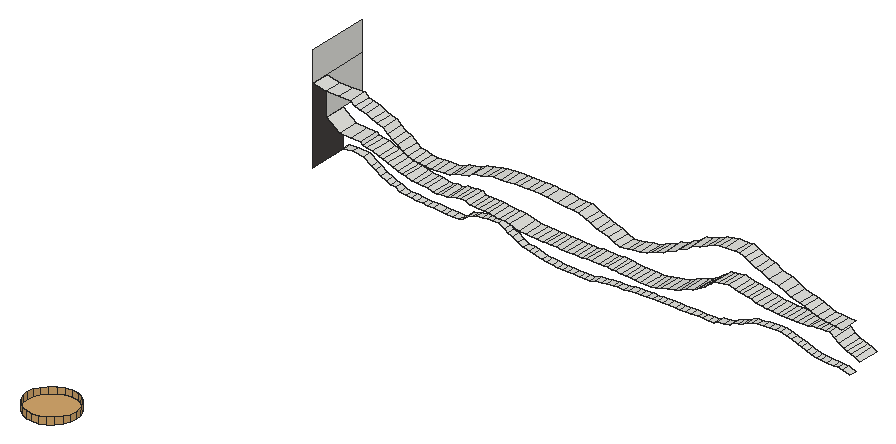
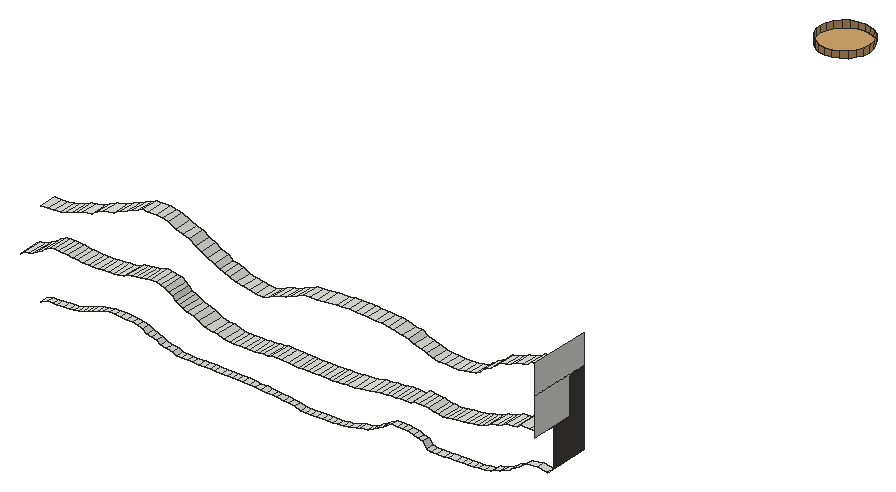
# SketchUp Ruby script. Lengths in inches.
U = 1.inch
M = Sketchup.active_model
def pt(a) = Geom::Point3d.new(a.map { |v| v * U })
def face(e, loops, mat)
  f = e.add_face(loops[0].map { |a| pt(a) })
  loops[1..].each { |l| e.add_face(l.map { |a| pt(a) }).erase! }
  f.material = f.back_material = mat if mat
  f
end
# faces: each face lists its corners as indices into pts; further lists are holes
def faces(e, pts, list, mat = nil) = list.each { |f| face(e, (f[0].is_a?(Array) ? f : [f]).map { |l| l.map { |i| pts[i] } }, mat) }
# xy, xz, yz: faces in a plane at the given z, y or x. An outline is a flat list of corners, or four numbers for a rectangle; further outlines are holes
def ring(l) = l.size == 4 ? [[l[0], l[1]], [l[2], l[1]], [l[2], l[3]], [l[0], l[3]]] : l.each_slice(2).to_a
def flat(e, list, mat, &to3) = list.each { |f| face(e, (f[0].is_a?(Array) ? f : [f]).map { |l| ring(l).map { |u, v| to3.(u, v) } }, mat) }
def xy(e, z, list, mat = nil) = flat(e, list, mat) { |x, y| [x, y, z] }
def xz(e, y, list, mat = nil) = flat(e, list, mat) { |x, z| [x, y, z] }
def yz(e, x, list, mat = nil) = flat(e, list, mat) { |y, z| [x, y, z] }
def lines(e, pts, list) = list.each { |a, b| e.add_line(pt(pts[a]), pt(pts[b])) }
# prism: a flat outline (further loops are holes) pulled along v
def prism(e, loops, v, mat = nil)
  f = face(e, loops, mat); d = Geom::Vector3d.new(v.map { |x| x * U })
  f.pushpull(f.normal.samedirection?(d) ? d.length : -d.length)
end
def box(e, o, s, mat = nil) = prism(e, [[o, [o[0] + s[0], o[1], o[2]], [o[0] + s[0], o[1] + s[1], o[2]], [o[0], o[1] + s[1], o[2]]]], [0, 0, s[2]], mat)
def at(x, y, z, deg = 0) = Geom::Transformation.translation(pt([x, y, z])) * Geom::Transformation.rotation(ORIGIN, Z_AXIS, deg.degrees)
def axes(o, x, y, z) = Geom::Transformation.new([*x, 0, *y, 0, *z, 0, *pt(o).to_a, 1])
def part(name) = M.definitions.add(name)
# library, detail: a bought-in or finely detailed component or shape, given as its bounding box
def library(name, o, s) = part(name).tap { |d| box(d.entities, o, s) }
def detail(e, o, s) = box(e.add_group.entities, o, s)
def put(e, d, t, mat = nil) = e.add_instance(d, t).tap { |i| i.material = mat if mat }
def group(e, t, mat = nil) = e.add_group.tap { |g| g.transformation = t; g.material = mat if mat }.entities
root = M.entities
M.materials.add("[Field Square Tile]").color = [211, 167, 108]
M.materials.add("[Granite Tile]1").color = [68, 65, 63]
xy(root,237.65,[[282.08,565.74,282.77,566.68],[282.77,565.74,283.39,566.68]])
xy(root,238.33,[[291.18,565.74,291.73,566.68],[291.73,565.74,292.41,566.68]])
xy(root,238.34,[[293.09,565.74,294.02,566.68],[294.02,565.74,294.51,566.68],[294.51,565.74,295.27,566.68],[295.27,565.74,295.9,566.68],[295.9,565.74,296.65,566.68],
  [296.65,565.74,297.27,566.68],[297.27,565.74,298.04,566.68],[298.04,565.74,298.66,566.68]])
xy(root,241.52,[[252.78,561.05,252.84,566.68]])
xy(root,241.68,[[283.28,563.18,283.87,565.74]])
xy(root,241.75,[[285.63,563.18,286.5,565.74],[286.5,563.18,287.12,565.74],[287.12,563.18,287.63,565.74]])
xy(root,250.6875,[[273.1,492.27,272.31,492.375,271.57,492.68,270.93,493.17,270.45,493.8,270.14,494.54,270.04,495.33,270.14,496.125,270.45,496.86,270.93,497.5,271.57,497.98,272.31,498.29,273.1,498.39,273.89,498.29,274.63,497.98,275.26,497.5,275.75,496.86,276.06,496.125,276.16,495.33,276.06,494.54,275.75,493.8,275.26,493.17,274.63,492.68,273.89,492.375]],"[Field Square Tile]")
xz(root,561.05,[[252.78,241.52,252.84,251.5]])
yz(root,252.84,[[563.18,246.2,568.68,250.88],[561.05,250.88,568.68,254.5]])
yz(root,252.84,[[561.05,241.52,565.74,241.52,565.74,246.2,563.18,246.2,563.18,250.88,561.05,250.88]],"[Granite Tile]1")
p = [[283.39,565.74,237.65],[283.39,566.68,237.65],[284.06,566.68,237.89],[284.06,565.74,237.89],[278.72,565.74,237.76],[278.72,566.68,237.76],
  [279.43,566.68,237.71],[279.43,565.74,237.71],[280.04,566.68,237.68],[280.04,565.74,237.68],[280.64,566.68,237.67],[280.64,565.74,237.67],
  [281.39,566.68,237.66],[281.39,565.74,237.66],[282.08,566.68,237.65],[282.08,565.74,237.65],[277.37,565.74,237.9],[277.37,566.68,237.9],
  [278.03,566.68,237.82],[278.03,565.74,237.82],[276.43,565.74,238.21],[276.43,566.68,238.21],[284.82,566.68,237.94],[284.82,565.74,237.94],
  [285.4375,566.68,237.98],[285.4375,565.74,237.98],[286.29,566.68,238.1],[286.29,565.74,238.1],[286.84,566.68,238.13],[286.84,565.74,238.13],
  [287.6,566.68,238.15],[287.6,565.74,238.15],[275.96,565.74,238.31],[275.96,566.68,238.31],[288.23,566.68,238.26],[288.23,565.74,238.26],
  [275.05,565.74,238.43],[275.05,566.68,238.43],[288.98,566.68,238.28],[288.98,565.74,238.28],[289.61,566.68,238.3],[289.61,565.74,238.3],
  [290.46,566.68,238.32],[290.46,565.74,238.32],[291.18,566.68,238.33],[291.18,565.74,238.33],[292.41,565.74,238.33],[292.41,566.68,238.33],
  [293.09,566.68,238.34],[293.09,565.74,238.34],[298.66,565.74,238.34],[298.66,566.68,238.34],[299.17,566.68,238.59],[299.17,565.74,238.59],
  [274.4,565.74,238.74],[274.4,566.68,238.74],[314.69,565.74,238.78],[314.69,566.68,238.78],[315.47,566.68,238.43],[315.47,565.74,238.43],
  [299.99,566.68,238.72],[299.99,565.74,238.72],[273.82,565.74,239.11],[273.82,566.68,239.11],[300.68,566.68,238.86],[300.68,565.74,238.86],
  [264.03,565.74,238.92],[264.03,566.68,238.92],[265.07,566.68,238.82],[265.07,565.74,238.82],[265.58,566.68,238.8],[265.58,565.74,238.8],
  [266.45,566.68,238.79],[266.45,565.74,238.79],[267.19,566.68,238.77],[267.19,565.74,238.77],[267.72,566.68,238.9375],[267.72,565.74,238.9375],
  [311.97,565.74,238.875],[311.97,566.68,238.875],[312.72,566.68,238.83],[312.72,565.74,238.83],[313.48,566.68,238.8],[313.48,565.74,238.8],
  [314.02,566.68,238.79],[314.02,565.74,238.79],[261.94,565.74,238.97],[261.94,566.68,238.97],[262.64,566.68,238.94],[262.64,565.74,238.94],
  [263.34,566.68,238.93],[263.34,565.74,238.93],[268.28,566.68,239.55],[268.28,565.74,239.55],[301.19,566.68,239.18],[301.19,565.74,239.18],
  [310.82,565.74,239.04],[310.82,566.68,239.04],[311.4,566.68,238.94],[311.4,565.74,238.94],[260.57,565.74,239.09],[260.57,566.68,239.09],
  [261.26,566.68,239.03],[261.26,565.74,239.03],[310.16,565.74,239.29],[310.16,566.68,239.29],[259.79,565.74,239.19],[259.79,566.68,239.19],
  [273.24,565.74,239.38],[273.24,566.68,239.38],[259.28,565.74,239.52],[259.28,566.68,239.52],[301.78,566.68,239.35],[301.78,565.74,239.35],
  [309.58,565.74,239.53],[309.58,566.68,239.53],[272.78,565.74,239.71],[272.78,566.68,239.71],[302.34,566.68,239.52],[302.34,565.74,239.52],
  [258.72,565.74,239.64],[258.72,566.68,239.64],[302.89,566.68,239.85],[302.89,565.74,239.85],[309.05,565.74,239.7],[309.05,566.68,239.7],
  [258.27,565.74,239.86],[258.27,566.68,239.86],[268.86,566.68,239.69],[268.86,565.74,239.69],[269.41,566.68,239.88],[269.41,565.74,239.88],
  [272.08,565.74,240.11],[272.08,566.68,240.11],[308.36,565.74,239.92],[308.36,566.68,239.92],[303.53,566.68,240.03],[303.53,565.74,240.03],
  [257.48,565.74,240.2],[257.48,566.68,240.2],[270.14,566.68,239.99],[270.14,565.74,239.99],[307.73,565.74,240.11],[307.73,566.68,240.11],
  [270.73,566.68,240.05],[270.73,565.74,240.05],[271.39,566.68,240.09],[271.39,565.74,240.09],[304.1875,566.68,240.12],[304.1875,565.74,240.12],
  [304.86,566.68,240.19],[304.86,565.74,240.19],[306.95,565.74,240.27],[306.95,566.68,240.27],[256.88,565.74,240.59],[256.88,566.68,240.59],
  [305.625,566.68,240.23],[305.625,565.74,240.23],[306.33,566.68,240.25],[306.33,565.74,240.25],[256.34,565.74,240.85],[256.34,566.68,240.85],
  [255.32,565.74,241.55],[255.32,566.68,241.55],[289.26,563.18,241.57],[289.26,565.74,241.57],[289.8,565.74,241.53],[289.8,563.18,241.53],
  [290.42,565.74,241.51],[290.42,563.18,241.51],[290.97,565.74,241.49],[290.97,563.18,241.49],[291.67,565.74,241.48],[291.67,563.18,241.48],
  [292.33,565.74,241.47],[292.33,563.18,241.47],[292.9,565.74,241.46],[292.9,563.18,241.46],[293.61,565.74,241.6],[293.61,563.18,241.6],
  [252.84,565.74,241.52],[252.84,566.68,241.52],[254.05,566.68,241.69],[254.05,565.74,241.69],[288.65,563.18,241.66],[288.65,565.74,241.66],
  [294.34,565.74,241.85],[294.34,563.18,241.85],[279.62,563.18,241.75],[279.62,565.74,241.75],[280.07,565.74,241.74],[280.07,563.18,241.74],
  [280.62,565.74,241.72],[280.62,563.18,241.72],[281.25,565.74,241.71],[281.25,563.18,241.71],[281.88,565.74,241.7],[281.88,563.18,241.7],
  [282.61,565.74,241.69],[282.61,563.18,241.69],[283.28,565.74,241.68],[283.28,563.18,241.68],[283.87,563.18,241.68],[283.87,565.74,241.68],
  [284.36,565.74,241.67],[284.36,563.18,241.67],[285.0625,565.74,241.74],[285.0625,563.18,241.74],[285.63,565.74,241.75],[285.63,563.18,241.75],
  [287.63,563.18,241.75],[287.63,565.74,241.75],[288.12,565.74,241.67],[288.12,563.18,241.67],[277.43,563.18,241.89],[277.43,565.74,241.89],
  [278.25,565.74,241.83],[278.25,563.18,241.83],[278.85,565.74,241.78],[278.85,563.18,241.78],[295.01,565.74,241.91],[295.01,563.18,241.91],
  [276.66,563.18,241.96],[276.66,565.74,241.96],[295.91,565.74,242.1],[295.91,563.18,242.1],[275.49,563.18,242.24],[275.49,565.74,242.24],
  [296.68,565.74,242.46],[296.68,563.18,242.46],[274.82,563.18,242.34],[274.82,565.74,242.34],[318.29,563.18,242.51],[318.29,565.74,242.51],
  [318.8,565.74,242.21],[318.8,563.18,242.21],[274.16,563.18,242.38],[274.16,565.74,242.38],[273.5,563.18,242.48],[273.5,565.74,242.48],
  [265.32,563.18,242.68],[265.32,565.74,242.68],[265.99,565.74,242.51],[265.99,563.18,242.51],[266.51,565.74,242.46],[266.51,563.18,242.46],
  [267.05,565.74,242.58],[267.05,563.18,242.58],[272.86,563.18,242.57],[272.86,565.74,242.57],[297.38,565.74,242.78],[297.38,563.18,242.78],
  [317.7,563.18,242.68],[317.7,565.74,242.68],[267.68,565.74,242.57],[267.68,563.18,242.57],[268.31,565.74,242.81],[268.31,563.18,242.81],
  [270.08,563.18,242.92],[270.08,565.74,242.92],[270.51,565.74,242.625],[270.51,563.18,242.625],[271.12,565.74,242.65],[271.12,563.18,242.65],
  [271.67,565.74,242.62],[271.67,563.18,242.62],[272.3,565.74,242.58],[272.3,563.18,242.58],[263.97,563.18,242.78],[263.97,565.74,242.78],
  [264.78,565.74,242.73],[264.78,563.18,242.73],[317.2,563.18,242.875],[317.2,565.74,242.875],[262.67,563.18,243.06],[262.67,565.74,243.06],
  [263.39,565.74,242.85],[263.39,563.18,242.85],[268.88,565.74,242.86],[268.88,563.18,242.86],[298.15,565.74,242.97],[298.15,563.18,242.97],
  [269.44,565.74,242.89],[269.44,563.18,242.89],[316.81,563.18,243.09],[316.81,565.74,243.09],[298.68,565.74,243.23],[298.68,563.18,243.23],
  [261.6,563.18,243.3],[261.6,565.74,243.3],[262.1875,565.74,243.14],[262.1875,563.18,243.14],[316.2,563.18,243.43],[316.2,565.74,243.43],
  [299.08,565.74,243.48],[299.08,563.18,243.48],[260.96,563.18,243.48],[260.96,565.74,243.48],[315.66,563.18,243.8],[315.66,565.74,243.8],
  [260.44,563.18,243.79],[260.44,565.74,243.79],[299.6,565.74,243.72],[299.6,563.18,243.72],[299.9375,565.74,244.12],[299.9375,563.18,244.12],
  [259.78,563.18,243.95],[259.78,565.74,243.95],[315.06,563.18,244.18],[315.06,565.74,244.18],[259.26,563.18,244.11],[259.26,565.74,244.11],
  [307.88,563.18,243.99],[307.88,565.74,243.99],[308.6,565.74,243.95],[308.6,563.18,243.95],[309.1,565.74,243.93],[309.1,563.18,243.93],
  [309.79,565.74,243.91],[309.79,563.18,243.91],[310.36,565.74,243.89],[310.36,563.18,243.89],[311.06,565.74,243.88],[311.06,563.18,243.88],
  [311.71,565.74,243.94],[311.71,563.18,243.94],[312.35,565.74,243.95],[312.35,563.18,243.95],[312.91,565.74,244.1],[312.91,563.18,244.1],
  [306.7,563.18,244.11],[306.7,565.74,244.11],[307.26,565.74,244.04],[307.26,563.18,244.04],[258.59,563.18,244.41],[258.59,565.74,244.41],
  [300.41,565.74,244.39],[300.41,563.18,244.39],[305.95,563.18,244.25],[305.95,565.74,244.25],[313.54,565.74,244.13],[313.54,563.18,244.13],
  [314.02,565.74,244.15],[314.02,563.18,244.15],[314.54,565.74,244.17],[314.54,563.18,244.17],[305.49,563.18,244.51],[305.49,565.74,244.51],
  [257.83,563.18,244.54],[257.83,565.74,244.54],[300.89,565.74,244.73],[300.89,563.18,244.73],[257.27,563.18,244.61],[257.27,565.74,244.61],
  [304.34,563.18,244.67],[304.34,565.74,244.67],[304.95,565.74,244.55],[304.95,563.18,244.55],[257.05,563.18,244.92],[257.05,565.74,244.92],
  [301.375,565.74,244.87],[301.375,563.18,244.87],[303.29,563.18,244.81],[303.29,565.74,244.81],[303.86,565.74,244.7],[303.86,563.18,244.7],
  [302.64,563.18,245.01],[302.64,565.74,245.01],[254.41,563.18,244.96],[254.41,565.74,244.96],[255.8,565.74,244.9375],[255.8,563.18,244.9375],
  [301.96,565.74,244.95],[301.96,563.18,244.95],[252.84,563.18,246.2],[252.84,565.74,246.2],[290.09,561.05,246.35],[290.09,563.18,246.35],
  [290.86,563.18,246.05],[290.86,561.05,246.05],[291.76,563.18,246.13],[291.76,561.05,246.13],[292.47,563.18,246.29],[292.47,561.05,246.29],
  [293.27,563.18,246.41],[293.27,561.05,246.41],[289.48,561.05,246.66],[289.48,563.18,246.66],[294.18,563.18,246.55],[294.18,561.05,246.55],
  [265.9,561.05,246.62],[265.9,563.18,246.62],[266.64,563.18,246.54],[266.64,561.05,246.54],[267.42,563.18,246.51],[267.42,561.05,246.51],
  [268.2,563.18,246.58],[268.2,561.05,246.58],[317.39,561.05,246.59],[317.39,563.18,246.59],[318.28,563.18,246.55],[318.28,561.05,246.55],
  [265.24,561.05,246.73],[265.24,563.18,246.73],[269,563.18,246.59],[269,561.05,246.59],[269.8,563.18,246.69],[269.8,561.05,246.69],
  [294.91,563.18,246.92],[294.91,561.05,246.92],[316.68,561.05,246.66],[316.68,563.18,246.66],[264.52,561.05,246.88],[264.52,563.18,246.88],
  [270.51,563.18,247.03],[270.51,561.05,247.03],[288.625,561.05,246.94],[288.625,563.18,246.94],[315.89,561.05,246.75],[315.89,563.18,246.75],
  [315.2,561.05,246.95],[315.2,563.18,246.95],[263.97,561.05,247.25],[263.97,563.18,247.25],[287.94,561.05,247.08],[287.94,563.18,247.08],
  [295.52,563.18,247.12],[295.52,561.05,247.12],[271.2,563.18,247.2],[271.2,561.05,247.2],[314.39,561.05,247.25],[314.39,563.18,247.25],
  [287.26,561.05,247.46],[287.26,563.18,247.46],[296.2,563.18,247.31],[296.2,561.05,247.31],[272.17,563.18,247.39],[272.17,561.05,247.39],
  [313.71,561.05,247.53],[313.71,563.18,247.53],[263.33,561.05,247.72],[263.33,563.18,247.72],[296.77,563.18,247.71],[296.77,561.05,247.71],
  [272.8,563.18,247.78],[272.8,561.05,247.78],[286.63,561.05,247.66],[286.63,563.18,247.66],[313.13,561.05,247.66],[313.13,563.18,247.66],
  [262.68,561.05,248.07],[262.68,563.18,248.07],[285.79,561.05,248.08],[285.79,563.18,248.08],[297.7,563.18,248.03],[297.7,561.05,248.03],
  [312,561.05,247.9],[312,563.18,247.9],[273.58,563.18,247.89],[273.58,561.05,247.89],[274.58,563.18,248.18],[274.58,561.05,248.18],
  [311.4,561.05,248.26],[311.4,563.18,248.26],[298.41,563.18,248.46],[298.41,561.05,248.46],[262.05,561.05,248.51],[262.05,563.18,248.51],
  [284.17,561.05,248.15],[284.17,563.18,248.15],[284.99,563.18,248.11],[284.99,561.05,248.11],[275.22,563.18,248.29],[275.22,561.05,248.29],
  [283.14,561.05,248.28],[283.14,563.18,248.28],[276.11,563.18,248.35],[276.11,561.05,248.35],[281.74,561.05,248.39],[281.74,563.18,248.39],
  [310.49,561.05,248.69],[310.49,563.18,248.69],[276.84,563.18,248.4],[276.84,561.05,248.4],[277.83,563.18,248.4375],[277.83,561.05,248.4375],
  [278.49,563.18,248.46],[278.49,561.05,248.46],[281.01,561.05,248.49],[281.01,563.18,248.49],[261.56,561.05,249.01],[261.56,563.18,249.01],
  [279.38,563.18,248.47],[279.38,561.05,248.47],[280.12,563.18,248.48],[280.12,561.05,248.48],[299.19,563.18,248.82],[299.19,561.05,248.82],
  [309.27,561.05,248.95],[309.27,563.18,248.95],[299.91,563.18,249.37],[299.91,561.05,249.37],[308.38,561.05,249.46],[308.38,563.18,249.46],
  [260.79,561.05,249.2],[260.79,563.18,249.2],[260.12,561.05,249.41],[260.12,563.18,249.41],[259.45,561.05,249.8],[259.45,563.18,249.8],
  [300.7,563.18,249.5625],[300.7,561.05,249.5625],[307.62,561.05,249.68],[307.62,563.18,249.68],[301.6,563.18,249.9],[301.6,561.05,249.9],
  [306.96,561.05,250.0625],[306.96,563.18,250.0625],[258.65,561.05,249.97],[258.65,563.18,249.97],[302.52,563.18,250.35],[302.52,561.05,250.35],
  [258.04,561.05,250.15],[258.04,563.18,250.15],[257.51,561.05,250.55],[257.51,563.18,250.55],[306.27,561.05,250.32],[306.27,563.18,250.32],
  [303.18,563.18,250.49],[303.18,561.05,250.49],[305.65,561.05,250.61],[305.65,563.18,250.61],[252.84,561.05,250.88],[252.84,563.18,250.88],
  [254.43,563.18,250.53],[254.43,561.05,250.53],[256.05,563.18,250.54],[256.05,561.05,250.54],[303.99,563.18,250.6],[303.99,561.05,250.6],
  [305.01,563.18,250.58],[305.01,561.05,250.58],[273.1,492.27,251.5],[272.31,492.375,251.5],[272.31,492.375,250.6875],[273.1,492.27,250.6875],
  [273.89,492.375,251.5],[273.89,492.375,250.6875],[271.57,492.68,251.5],[271.57,492.68,250.6875],[274.63,492.68,251.5],[274.63,492.68,250.6875],
  [270.93,493.17,251.5],[270.93,493.17,250.6875],[275.26,493.17,251.5],[275.26,493.17,250.6875],[270.45,493.8,251.5],[270.45,493.8,250.6875],
  [275.75,493.8,251.5],[275.75,493.8,250.6875],[270.14,494.54,251.5],[270.14,494.54,250.6875],[276.06,494.54,251.5],[276.06,494.54,250.6875],
  [270.04,495.33,251.5],[270.04,495.33,250.6875],[276.16,495.33,251.5],[276.16,495.33,250.6875],[270.14,496.125,251.5],[270.14,496.125,250.6875],
  [276.06,496.125,251.5],[276.06,496.125,250.6875],[270.45,496.86,251.5],[270.45,496.86,250.6875],[275.75,496.86,251.5],[275.75,496.86,250.6875],
  [270.93,497.5,251.5],[270.93,497.5,250.6875],[275.26,497.5,251.5],[275.26,497.5,250.6875],[271.57,497.98,251.5],[271.57,497.98,250.6875],
  [274.63,497.98,251.5],[274.63,497.98,250.6875],[272.31,498.29,251.5],[272.31,498.29,250.6875],[273.89,498.29,251.5],[273.89,498.29,250.6875],
  [273.1,498.39,251.5],[273.1,498.39,250.6875]]
faces(root,p,[[0,1,2,3],[4,5,6,7],[7,6,8,9],[9,8,10,11],[11,10,12,13],[13,12,14,15],[16,17,18,19],[19,18,5,4],
  [20,21,17,16],[3,2,22,23],[23,22,24,25],[25,24,26,27],[27,26,28,29],[29,28,30,31],[32,33,21,20],[31,30,34,35],
  [36,37,33,32],[35,34,38,39],[39,38,40,41],[41,40,42,43],[43,42,44,45],[46,47,48,49],[50,51,52,53],[54,55,37,36],
  [56,57,58,59],[53,52,60,61],[62,63,55,54],[61,60,64,65],[66,67,68,69],[69,68,70,71],[71,70,72,73],[73,72,74,75],
  [75,74,76,77],[78,79,80,81],[81,80,82,83],[83,82,84,85],[85,84,57,56],[86,87,88,89],[89,88,90,91],[91,90,67,66],
  [77,76,92,93],[65,64,94,95],[96,97,98,99],[99,98,79,78],[100,101,102,103],[103,102,87,86],[104,105,97,96],[106,107,101,100],
  [108,109,63,62],[110,111,107,106],[95,94,112,113],[114,115,105,104],[116,117,109,108],[113,112,118,119],[120,121,111,110],[119,118,122,123],
  [124,125,115,114],[126,127,121,120],[93,92,128,129],[129,128,130,131],[132,133,117,116],[134,135,125,124],[123,122,136,137],[138,139,127,126],
  [131,130,140,141],[142,143,135,134],[141,140,144,145],[145,144,146,147],[137,136,148,149],[147,146,133,132],[149,148,150,151],[152,153,143,142],
  [154,155,139,138],[151,150,156,157],[157,156,158,159],[159,158,153,152],[160,161,155,154],[162,163,161,160],[164,165,166,167],[167,166,168,169],
  [169,168,170,171],[171,170,172,173],[173,172,174,175],[175,174,176,177],[177,176,178,179],[180,181,182,183],[184,185,165,164],[179,178,186,187],
  [183,182,163,162],[188,189,190,191],[191,190,192,193],[193,192,194,195],[195,194,196,197],[197,196,198,199],[199,198,200,201],[202,203,204,205],
  [205,204,206,207],[207,206,208,209],[210,211,212,213],[213,212,185,184],[214,215,216,217],[217,216,218,219],[219,218,189,188],[187,186,220,221],
  [222,223,215,214],[221,220,224,225],[226,227,223,222],[225,224,228,229],[230,231,227,226],[232,233,234,235],[236,237,231,230],[238,239,237,236],
  [240,241,242,243],[243,242,244,245],[245,244,246,247],[248,249,239,238],[229,228,250,251],[252,253,233,232],[247,246,254,255],[255,254,256,257],
  [258,259,260,261],[261,260,262,263],[263,262,264,265],[265,264,266,267],[267,266,249,248],[268,269,270,271],[271,270,241,240],[272,273,253,252],
  [274,275,276,277],[277,276,269,268],[257,256,278,279],[251,250,280,281],[279,278,282,283],[283,282,259,258],[284,285,273,272],[281,280,286,287],
  [288,289,290,291],[291,290,275,274],[292,293,285,284],[287,286,294,295],[296,297,289,288],[298,299,293,292],[300,301,297,296],[295,294,302,303],
  [303,302,304,305],[306,307,301,300],[308,309,299,298],[310,311,307,306],[312,313,314,315],[315,314,316,317],[317,316,318,319],[319,318,320,321],
  [321,320,322,323],[323,322,324,325],[325,324,326,327],[327,326,328,329],[330,331,332,333],[333,332,313,312],[334,335,311,310],[305,304,336,337],
  [338,339,331,330],[329,328,340,341],[341,340,342,343],[343,342,344,345],[345,344,309,308],[346,347,339,338],[348,349,335,334],[337,336,350,351],
  [352,353,349,348],[354,355,356,357],[357,356,347,346],[358,359,353,352],[351,350,360,361],[362,363,364,365],[365,364,355,354],[366,367,363,362],
  [368,369,370,371],[371,370,359,358],[361,360,372,373],[373,372,367,366],[374,375,369,368],[376,377,378,379],[379,378,380,381],[381,380,382,383],
  [383,382,384,385],[386,387,377,376],[385,384,388,389],[390,391,392,393],[393,392,394,395],[395,394,396,397],[398,399,400,401],[402,403,391,390],
  [397,396,404,405],[405,404,406,407],[389,388,408,409],[410,411,399,398],[412,413,403,402],[407,406,414,415],[416,417,387,386],[418,419,411,410],
  [420,421,419,418],[422,423,413,412],[424,425,417,416],[409,408,426,427],[415,414,428,429],[430,431,421,420],[432,433,425,424],[427,426,434,435],
  [429,428,436,437],[438,439,431,430],[440,441,423,422],[435,434,442,443],[437,436,444,445],[446,447,433,432],[448,449,439,438],[450,451,441,440],
  [452,453,447,446],[443,442,454,455],[456,457,449,448],[445,444,458,459],[459,458,460,461],[462,463,457,456],[455,454,464,465],[466,467,451,450],
  [468,469,470,471],[471,470,453,452],[461,460,472,473],[474,475,469,468],[473,472,476,477],[478,479,475,474],[480,481,463,462],[477,476,482,483],
  [483,482,484,485],[485,484,486,487],[488,489,479,478],[490,491,467,466],[487,486,492,493],[493,492,494,495],[495,494,489,488],[465,464,496,497],
  [498,499,481,480],[497,496,500,501],[502,503,499,498],[504,505,491,490],[506,507,505,504],[508,509,507,506],[501,500,510,511],[512,513,503,502],
  [511,510,514,515],[516,517,513,512],[518,519,509,508],[515,514,520,521],[522,523,519,518],[524,525,523,522],[526,527,517,516],[521,520,528,529],
  [530,531,527,526],[532,533,534,535],[535,534,536,537],[537,536,525,524],[529,528,538,539],[539,538,540,541],[541,540,531,530]])
faces(root,p,[[542,543,544,545],[546,542,545,547],[543,548,549,544],[550,546,547,551],[548,552,553,549],[554,550,551,555],[552,556,557,553],[558,554,555,559],
  [556,560,561,557],[562,558,559,563],[560,564,565,561],[566,562,563,567],[564,568,569,565],[570,566,567,571],[568,572,573,569],[574,570,571,575],
  [572,576,577,573],[578,574,575,579],[576,580,581,577],[582,578,579,583],[580,584,585,581],[586,582,583,587],[584,588,589,585],[588,586,587,589]],"[Field Square Tile]")
